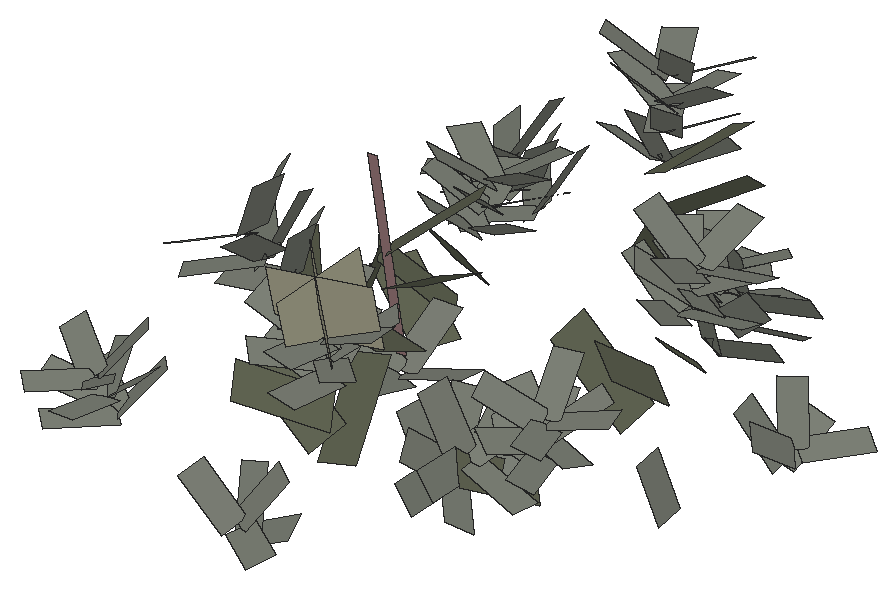
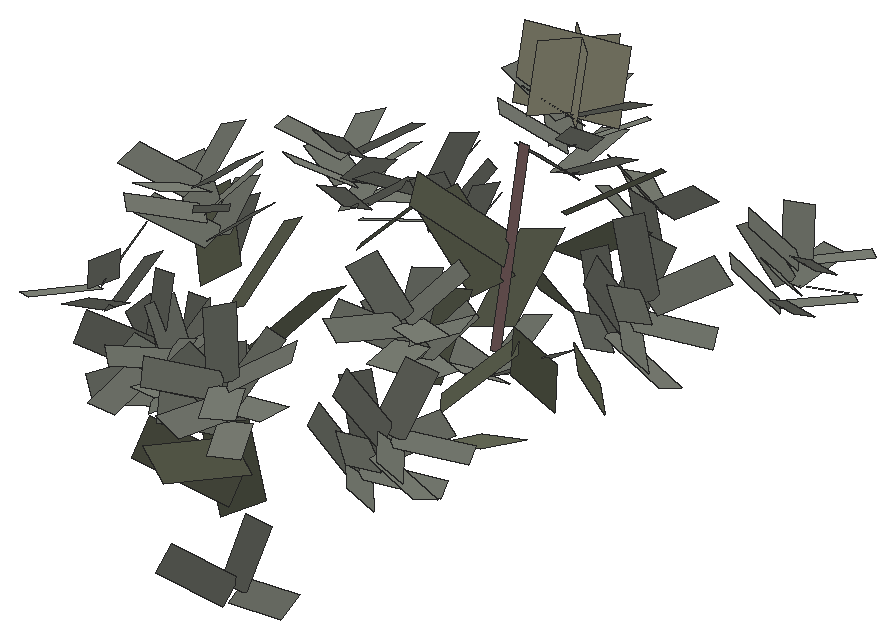
# SketchUp Ruby script. Lengths in inches.
U = 1.inch
M = Sketchup.active_model
def pt(a) = Geom::Point3d.new(a.map { |v| v * U })
def face(e, loops, mat)
  f = e.add_face(loops[0].map { |a| pt(a) })
  loops[1..].each { |l| e.add_face(l.map { |a| pt(a) }).erase! }
  f.material = f.back_material = mat if mat
  f
end
# faces: each face lists its corners as indices into pts; further lists are holes
def faces(e, pts, list, mat = nil) = list.each { |f| face(e, (f[0].is_a?(Array) ? f : [f]).map { |l| l.map { |i| pts[i] } }, mat) }
# xy, xz, yz: faces in a plane at the given z, y or x. An outline is a flat list of corners, or four numbers for a rectangle; further outlines are holes
def ring(l) = l.size == 4 ? [[l[0], l[1]], [l[2], l[1]], [l[2], l[3]], [l[0], l[3]]] : l.each_slice(2).to_a
def flat(e, list, mat, &to3) = list.each { |f| face(e, (f[0].is_a?(Array) ? f : [f]).map { |l| ring(l).map { |u, v| to3.(u, v) } }, mat) }
def xy(e, z, list, mat = nil) = flat(e, list, mat) { |x, y| [x, y, z] }
def xz(e, y, list, mat = nil) = flat(e, list, mat) { |x, z| [x, y, z] }
def yz(e, x, list, mat = nil) = flat(e, list, mat) { |y, z| [x, y, z] }
def lines(e, pts, list) = list.each { |a, b| e.add_line(pt(pts[a]), pt(pts[b])) }
# prism: a flat outline (further loops are holes) pulled along v
def prism(e, loops, v, mat = nil)
  f = face(e, loops, mat); d = Geom::Vector3d.new(v.map { |x| x * U })
  f.pushpull(f.normal.samedirection?(d) ? d.length : -d.length)
end
def box(e, o, s, mat = nil) = prism(e, [[o, [o[0] + s[0], o[1], o[2]], [o[0] + s[0], o[1] + s[1], o[2]], [o[0], o[1] + s[1], o[2]]]], [0, 0, s[2]], mat)
def at(x, y, z, deg = 0) = Geom::Transformation.translation(pt([x, y, z])) * Geom::Transformation.rotation(ORIGIN, Z_AXIS, deg.degrees)
def axes(o, x, y, z) = Geom::Transformation.new([*x, 0, *y, 0, *z, 0, *pt(o).to_a, 1])
def part(name) = M.definitions.add(name)
# library, detail: a bought-in or finely detailed component or shape, given as its bounding box
def library(name, o, s) = part(name).tap { |d| box(d.entities, o, s) }
def detail(e, o, s) = box(e.add_group.entities, o, s)
def put(e, d, t, mat = nil) = e.add_instance(d, t).tap { |i| i.material = mat if mat }
def group(e, t, mat = nil) = e.add_group.tap { |g| g.transformation = t; g.material = mat if mat }.entities
root = M.entities
M.materials.add("tak1dsfasd0f156w").color = [150, 118, 119]
M.materials.add("viburnumblaasdfas0df1w06d").color = [98, 102, 84]
M.materials.add("viburnumbladsadfasdfad0w122").color = [125, 129, 119]
M.materials.add("viburnumbloem2asdfas01vxc5016").color = [175, 173, 148]
c1 = part("Component\#315")
p = [[0.25,0,0],[2.05,0.01,0.35],[1.81,4.2,1.66],[0,4.19,1.3125]]
faces(c1.entities,p,[[0,1,2,3]],"viburnumbladsadfasdfad0w122")
c2 = part("viburnumblad2")
put(c2.entities,c1,axes([-19.23,-4.49,-32.18],[83.35428,0,0],[0,79.38502,0],[0,0,83.35428]))
c3 = part("Component\#314")
p = [[0.14,0,0],[2.58,0.05,0.25],[2.44,5.11,2.64],[0,5.05,2.39]]
faces(c3.entities,p,[[0,1,2,3]],"viburnumblaasdfas0df1w06d")
c4 = part("viburnumblad1\#2")
put(c4.entities,c3,axes([-37.25,6.23,19.31],[75.98784,0,0],[0,65.50676,0],[0,0,75.98784]))
c5 = part("Component\#336")
p = [[6.03,1.45,4.43],[5.85,2.68,0.17],[0,1.22,0],[0.18,0,4.25]]
faces(c5.entities,p,[[0,1,2,3]],"viburnumbloem2asdfas01vxc5016")
c6 = part("Component\#334")
p = [[0.16,3.84,5.17],[0,4.97,1.27],[3.78,1.125,0],[3.9375,0,3.9]]
faces(c6.entities,p,[[0,1,2,3]],"viburnumbloem2asdfas01vxc5016")
c7 = part("Component\#335")
p = [[1.35,5.21,5.35],[1.19,6.33,1.45],[0,1.125,0],[0.16,0,3.9]]
faces(c7.entities,p,[[0,1,2,3]],"viburnumbloem2asdfas01vxc5016")
c8 = part("Component\#337")
p = [[0.6,0,12.07],[1.51,1.22,0.03],[0.91,1.23,0],[0,0,12.04]]
faces(c8.entities,p,[[0,1,2,3]],"tak1dsfasd0f156w")
put(root,c2,axes([2210.91,246.79,41.88],[-0.00636,-0.00796,-0.00575],[0.0099,-0.00571,-0.00294],[-0.00097,-0.00646,0.0087]))
put(root,c2,axes([2209.49,245.54,40.99],[0.00636,0.00796,0.00575],[-0.00984,0.00398,0.00495],[0.00146,-0.00765,0.00773]))
put(root,c2,axes([2209.42,246.71,41.875],[0.00995,-0.00489,-0.00397],[0.00634,0.00703,0.00672],[-0.00053,-0.00802,0.00751]))
put(root,c2,axes([2209.95,247.92,40.99],[0.00254,-0.00908,-0.00688],[0.01053,0.00118,0.00207],[-0.00116,-0.00732,0.00806]))
put(root,c2,axes([2209.29,246.93,40.29],[0.01153,0.00217,0.00126],[-0.00261,0.00855,0.00823],[0.00055,-0.00816,0.00738]))
put(root,c2,axes([2197.875,249.31,44.43],[-0.00773,0.00806,0.00054],[-0.00787,-0.00734,-0.00302],[-0.00183,-0.00247,0.01075]))
put(root,c2,axes([2198.58,250.46,43.45],[-0.01083,0.00076,-0.00267],[-0.00024,-0.01097,-0.00215],[-0.00276,-0.00202,0.01064]))
put(root,c2,axes([2198.09,250.62,44.91],[-0.00759,-0.00699,-0.00431],[0.00733,-0.00841,0.00072],[-0.00369,-0.00233,0.01029]))
put(root,c2,axes([2198.58,250.47,41.96],[-0.00742,0.00774,0.00052],[-0.0085,-0.00793,-0.00326],[-0.00183,-0.00247,0.01075]))
put(root,c2,axes([2197.65,249.76,42.95],[-0.0001,0.01064,0.00343],[-0.01164,0.00037,-0.00146],[-0.00143,-0.00341,0.01055]))
put(root,c2,axes([2197.74,251.62,43.6],[0.0001,-0.01064,-0.00343],[0.01052,-0.00118,0.00394],[-0.00407,-0.00322,0.0099]))
put(root,c2,axes([2211.68,253.05,50.16],[-0.01255,0.00027,0.0006],[-0.00036,-0.0124,-0.00196],[0.00055,-0.00198,0.01239]))
put(root,c2,axes([2196.52,249.63,44.17],[0.00759,0.00699,0.00431],[-0.00801,0.0076,0.00179],[-0.00181,-0.0043,0.01016]))
put(root,c2,axes([2196.74,250.94,44.66],[0.00773,-0.00806,-0.00054],[0.0072,0.00653,0.00553],[-0.00368,-0.00417,0.0097]))
put(root,c2,axes([2196.68,250.64,42.96],[0.01083,-0.00076,0.00267],[-0.0004,0.00932,0.00428],[-0.00274,-0.00461,0.00981]))
put(root,c2,axes([2211.3,254.2,47.23],[-0.01204,0.00026,0.00058],[-0.00039,-0.0134,-0.00212],[0.00055,-0.00198,0.01239]))
put(root,c2,axes([2211.14,253.03,48.49],[-0.00857,0.00873,0.00287],[-0.00949,-0.00914,-0.00056],[0.00162,-0.00243,0.01222]))
put(root,c2,axes([2197.19,250.67,41.69],[0.00793,0.00729,0.0045],[-0.00721,0.00684,0.00161],[-0.00181,-0.0043,0.01016]))
put(root,c2,axes([2197.3,251.77,42.17],[0.00743,-0.00696,-0.00145],[0.0072,0.00653,0.00553],[-0.00282,-0.00502,0.00959]))
put(root,c2,axes([2211.3125,254.38,48.9],[-0.00917,-0.00834,-0.00202],[0.00857,-0.00908,-0.00138],[-0.00054,-0.00239,0.01232]))
put(root,c4,axes([2210.54,254.06,43.96],[-0.00623,0.01061,0.0062],[-0.01365,-0.00831,0.0005],[0.00356,-0.0051,0.0123]))
put(root,c5,axes([2207.86,251.38,49.92],[1.0472,0,0],[0,1.0472,0],[0,0,1.0472]))
put(root,c6,axes([2208.61,250.23,49.61],[1.0472,0,0],[0,1.0472,0],[0,0,1.0472]))
put(root,c2,axes([2210.35,252.2,49.97],[0.00042,0.01207,0.00346],[-0.01239,-0.00016,0.00207],[0.00203,-0.00348,0.0119]))
put(root,c7,axes([2210.11,249.6,49.53],[1.0472,0,0],[0,1.0472,0],[0,0,1.0472]))
put(root,c2,axes([2210.81,254.32,50.5625],[-0.00042,-0.01207,-0.00346],[0.01251,-0.00069,0.00087],[-0.00103,-0.00342,0.01205]))
put(root,c2,axes([2218.88,255.93,43.26],[-0.00894,0.00051,0.00882],[-0.00128,-0.01248,-0.00058],[0.00874,-0.00131,0.00893]))
put(root,c2,axes([2210.04,253.22,47.05],[0.00044,0.0126,0.00361],[-0.01115,-0.00014,0.00186],[0.00203,-0.00348,0.0119]))
put(root,c2,axes([2209.66,252.96,48.52],[0.00917,0.00834,0.00202],[-0.00775,0.00756,0.00397],[0.00155,-0.00451,0.01162]))
put(root,c2,axes([2216.625,256.45,41.18],[-0.00933,0.00053,0.0092],[-0.00115,-0.01124,-0.00052],[0.00874,-0.00131,0.00893]))
put(root,c2,axes([2217.64,257.13,42.53],[-0.00797,-0.00829,0.00506],[0.00596,-0.00975,-0.0066],[0.00788,-0.0017,0.00963]))
put(root,c2,axes([2217.44,255.69,42.25],[-0.00467,0.00901,0.00741],[-0.00631,-0.00787,0.00559],[0.00942,-0.00179,0.00811]))
put(root,c4,axes([2209.14,254.43,41.85],[0.00552,0.01118,0.00587],[-0.01458,0.00491,0.00435],[0.00124,-0.00686,0.01189]))
put(root,c2,axes([2209.48,253.47,50.375],[0.01255,-0.00027,-0.0006],[0.00048,0.01156,0.0049],[0.00045,-0.00492,0.01155]))
put(root,c2,axes([2209.73,254.65,49.04],[0.00857,-0.00873,-0.00287],[0.00926,0.00794,0.00351],[-0.00062,-0.00447,0.01173]))
put(root,c2,axes([2217.79,255.09,44.05],[0.00233,0.01223,0.00166],[-0.00783,0.00016,0.00982],[0.00954,-0.00286,0.00766]))
put(root,c2,axes([2209.25,254.24,47.47],[0.01143,0.00024,-0.0017],[0.00048,0.01156,0.0049],[0.0018,-0.00492,0.01142]))
put(root,c2,axes([2218.47,257.23,44.07],[-0.00233,-0.01223,-0.00166],[0.00991,-0.00085,-0.00768],[0.00736,-0.00274,0.0098]))
put(root,c2,axes([2215.78,255.66,41.89],[0.00119,0.01147,0.00076],[-0.00783,0.00016,0.00982],[0.00974,-0.00152,0.00779]))
put(root,c2,axes([2222.57,258.84,46.21],[-0.01096,-0.00354,0.00194],[0.00316,-0.01102,-0.00224],[0.00251,-0.00157,0.0113]))
put(root,c2,axes([2221.92,258.67,44.73],[-0.00975,0.0051,0.00392],[-0.00563,-0.0109,0.00018],[0.00356,-0.00165,0.01101]))
put(root,c4,axes([2220.57,259.39,40.65],[-0.00789,0.00746,0.00681],[-0.00938,-0.01142,0.00165],[0.00606,-0.00342,0.01077]))
put(root,c2,axes([2221.56,259.74,43.59],[-0.01053,-0.0034,0.00186],[0.00341,-0.01191,-0.00242],[0.00251,-0.00157,0.0113]))
put(root,c2,axes([2216.2,255.76,43.52],[0.00797,0.00829,-0.00506],[-0.00363,0.00868,0.00851],[0.00902,-0.0039,0.00783]))
put(root,c2,axes([2221.65,257.69,46.15],[-0.00283,0.01075,0.0036],[-0.01053,-0.00387,0.00326],[0.00419,-0.00245,0.01063]))
put(root,c2,axes([2216.68,257.3,43.5625],[0.00467,-0.00901,-0.00741],[0.00895,0.00789,-0.00395],[0.00748,-0.00381,0.00935]))
put(root,c2,axes([2217.38,256.39,44.86],[0.00894,-0.00051,-0.00882],[0.00335,0.0118,0.00272],[0.00817,-0.00429,0.00853]))
put(root,c2,axes([2221.71,259.91,45.14],[-0.00575,-0.0101,-0.00117],[0.01003,-0.00542,-0.00255],[0.00167,-0.00226,0.01134]))
put(root,c4,axes([2208.125,256.4,39.75],[0.0147,-0.00029,0.00242],[-0.00086,0.01575,0.00709],[-0.00232,-0.00615,0.01338]))
put(root,c2,axes([2220.74,258.5,43.52],[-0.00295,0.01122,0.00376],[-0.00948,-0.00348,0.00294],[0.00419,-0.00245,0.01063]))
put(root,c2,axes([2221.48,259.69,46.72],[0.00283,-0.01075,-0.0036],[0.01123,0.00316,-0.00059],[0.00152,-0.00332,0.0111]))
put(root,c2,axes([2220.65,258.16,44.91],[0.00575,0.0101,0.00117],[-0.00857,0.00432,0.00479],[0.00404,-0.00351,0.01039]))
put(root,c2,axes([2220.56,258.55,46.66],[0.01096,0.00354,-0.00194],[-0.00246,0.01032,0.00491],[0.0032,-0.00419,0.01042]))
put(root,c2,axes([2220.27,259.66,45.45],[0.00975,-0.0051,-0.00392],[0.00612,0.00977,0.00252],[0.00215,-0.00412,0.01072]))
put(root,c2,axes([2219.79,259.16,44.04],[0.00971,0.00365,-0.00281],[-0.00246,0.01032,0.00491],[0.00437,-0.00379,0.01015]))
put(root,c2,axes([2198.02,262.85,48.33],[-0.00996,0.00362,-0.00815],[-0.00316,-0.01285,-0.00186],[-0.00834,0.00054,0.01043]))
put(root,c2,axes([2199.18,264.05,47.21],[-0.00854,-0.00651,-0.00796],[0.00449,-0.01178,0.00482],[-0.00927,0.0004,0.00962]))
put(root,c4,axes([2207.59,265.23,42.92],[-0.0155,-0.00126,0.00308],[0.00163,-0.01831,0.00072],[0.00301,0.00088,0.01554]))
put(root,c2,axes([2198.72,262.5,46.66],[-0.00554,0.01163,-0.00356],[-0.00953,-0.00658,-0.00667],[-0.00756,-0.00023,0.01102]))
put(root,c2,axes([2226.6,262.48,39.98],[-0.00142,0.01147,0.00174],[-0.00575,-0.00222,0.00993],[0.01007,0.00035,0.00591]))
put(root,c2,axes([2197.51,264.4375,48.06],[-0.00212,-0.01282,-0.00311],[0.00883,-0.00372,0.00932],[-0.00981,-0.00058,0.00906]))
put(root,c2,axes([2207.35,265.27,40.98],[-0.01323,-0.00019,0.0019],[0.00023,-0.01336,0.00026],[0.00189,0.00029,0.01323]))
put(root,c2,axes([2199.55,264.8125,45.62],[-0.00096,-0.01167,-0.00375],[0.00883,-0.00372,0.00932],[-0.00998,-0.00196,0.00867]))
put(root,c2,axes([2199.27,262.74,44.98],[0.00203,0.01231,0.00299],[-0.01181,0.00375,-0.0074],[-0.00738,-0.00146,0.01104]))
put(root,c8,axes([2205.03,263.99,42.22],[1.0472,0,0],[0,1.0472,0],[0,0,1.0472]))
put(root,c2,axes([2197.8,264.57,46.03],[0.00554,-0.01163,0.00356],[0.00681,0.00581,0.00839],[-0.00964,-0.00181,0.00908]))
put(root,c4,axes([2206.57,266.31,45.8125],[-0.00531,-0.01357,0.00158],[0.01582,-0.00598,0.00178],[-0.00086,0.00203,0.01449]))
put(root,c2,axes([2205.98,264.28,41.08],[0,0.0133,0.00135],[-0.0129,-0.00035,0.00349],[0.0035,-0.0013,0.01283]))
put(root,c2,axes([2197.64,263.03,45.75],[0.00854,0.00651,0.00796],[-0.00689,0.01199,-0.00242],[-0.00792,-0.00244,0.01048]))
put(root,c2,axes([2196.33,263.88,46.99],[0.00996,-0.00362,0.00815],[0.00104,0.0126,0.00432],[-0.00886,-0.00258,0.00967]))
put(root,c2,axes([2206.38,266.625,41.26],[0,-0.0133,-0.00135],[0.01336,0.00003,-0.00028],[0.00028,-0.00135,0.01329]))
put(root,c2,axes([2198.63,264.28,44.64],[0.01039,-0.00378,0.00851],[0.00094,0.01134,0.00389],[-0.00886,-0.00258,0.00967]))
put(root,c4,axes([2200.69,263.9,41.91],[0.00849,0.00329,0.01149],[-0.00585,0.01597,-0.00025],[-0.01083,-0.00383,0.0091]))
put(root,c4,axes([2205.18,265.79,48.1],[0.00718,-0.01267,0.00168],[0.01433,0.00855,0.00326],[-0.00327,0.00004,0.01429]))
put(root,c4,axes([2202.2,265.49,40.29],[0.00719,-0.00894,0.00913],[0.00526,0.01343,0.009],[-0.01194,-0.00098,0.00844]))
put(root,c2,axes([2205.02,265.64,41.35],[0.01323,0.00019,-0.0019],[0.00023,0.01303,0.00294],[0.00189,-0.00295,0.0129]))
put(root,c4,axes([2220.42,270.45,41.85],[-0.01118,0.00552,0.00587],[-0.00491,-0.01458,0.00435],[0.00686,0.00124,0.01189]))
put(root,c4,axes([2220.79,271.85,43.96],[-0.01061,-0.00623,0.0062],[0.00831,-0.01365,0.0005],[0.0051,0.00356,0.0123]))
put(root,c2,axes([2221.63,271.35,47.05],[-0.0126,0.00044,0.00361],[0.00014,-0.01115,0.00186],[0.00348,0.00203,0.0119]))
put(root,c2,axes([2229.3125,270.79,40.99],[-0.00796,0.00636,0.00575],[-0.00398,-0.00984,0.00495],[0.00765,0.00146,0.00773]))
put(root,c2,axes([2222.65,271.66,49.97],[-0.01207,0.00042,0.00346],[0.00016,-0.01239,0.00207],[0.00348,0.00203,0.0119]))
put(root,c4,axes([2218.45,269.43,39.75],[0.00029,0.0147,0.00242],[-0.01575,-0.00086,0.00709],[0.00615,-0.00232,0.01338]))
put(root,c4,axes([2205.79,270.6,41.71],[-0.00837,0.01093,-0.00027],[-0.01213,-0.00903,0.00454],[0.00324,0.00308,0.01192]))
put(root,c2,axes([2221.89,270.97,48.52],[-0.00834,0.00917,0.00202],[-0.00756,-0.00775,0.00397],[0.00451,0.00155,0.01162]))
put(root,c2,axes([2221.82,272.45,48.49],[-0.00873,-0.00857,0.00287],[0.00914,-0.00949,-0.00056],[0.00243,0.00162,0.01222]))
put(root,c4,axes([2206.21,272.46,43.3],[-0.0135,0.00082,0.00242],[0.00046,-0.01443,0.00598],[0.00274,0.00585,0.01119]))
put(root,c2,axes([2227.92,270.6,40.29],[-0.00217,0.01153,0.00126],[-0.00855,-0.00261,0.00823],[0.00816,0.00055,0.00738]))
put(root,c2,axes([2220.61,270.56,47.47],[-0.00024,0.01143,-0.0017],[-0.01156,0.00048,0.0049],[0.00492,0.0018,0.01142]))
put(root,c2,axes([2221.39,270.79,50.375],[0.00027,0.01255,-0.0006],[-0.01156,0.00048,0.0049],[0.00492,0.00045,0.01155]))
put(root,c2,axes([2220.65,272.6,47.23],[-0.00026,-0.01204,0.00058],[0.0134,-0.00039,-0.00212],[0.00198,0.00055,0.01239]))
put(root,c4,axes([2204.2,269.65,39.48],[0.00652,0.01335,-0.00071],[-0.01553,0.00758,0.00028],[0.00058,0.00086,0.01356]))
put(root,c2,axes([2205.86,272.9,46.21],[-0.01136,0.00626,-0.00167],[-0.00561,-0.00886,0.00368],[0.00077,0.00497,0.01057]))
put(root,c2,axes([2221.8,272.99,50.16],[-0.00027,-0.01255,0.0006],[0.0124,-0.00036,-0.00196],[0.00198,0.00055,0.01239]))
put(root,c2,axes([2228.14,270.73,41.875],[0.00489,0.00995,-0.00397],[-0.00703,0.00634,0.00672],[0.00802,-0.00053,0.00751]))
put(root,c2,axes([2206.16,274.32,47.25],[-0.01214,-0.0031,0.00083],[0.00339,-0.01158,0.00463],[-0.0004,0.00512,0.01053]))
put(root,c2,axes([2206.1,273.9,48.91],[-0.01088,0.00599,-0.0016],[-0.00623,-0.00984,0.00409],[0.00077,0.00497,0.01057]))
put(root,c2,axes([2205.58,274.39,45.78],[-0.00603,-0.00996,0.00266],[0.01166,-0.00593,0.00316],[-0.00133,0.00444,0.01071]))
put(root,c2,axes([2220.2,271.04,49.04],[0.00873,0.00857,-0.00287],[-0.00794,0.00926,0.00351],[0.00447,-0.00062,0.01173]))
put(root,c2,axes([2226.93,271.26,40.99],[0.00908,0.00254,-0.00688],[-0.00118,0.01053,0.00207],[0.00732,-0.00116,0.00806]))
put(root,c2,axes([2228.0625,272.22,41.88],[0.00796,-0.00636,-0.00575],[0.00571,0.0099,-0.00294],[0.00646,-0.00097,0.0087]))
put(root,c2,axes([2220.47,272.62,48.9],[0.00834,-0.00917,-0.00202],[0.00908,0.00857,-0.00138],[0.00239,-0.00054,0.01232]))
put(root,c2,axes([2205.52,273.04,47.58],[-0.00325,0.01157,-0.00309],[-0.01106,-0.00241,0.00198],[0.00148,0.00409,0.01081]))
put(root,c2,axes([2205.96,275.41,48.5],[-0.00628,-0.01038,0.00277],[0.0108,-0.00549,0.00293],[-0.00133,0.00444,0.01071]))
put(root,c2,axes([2220.53,272.12,50.5625],[0.01207,-0.00042,-0.00346],[0.00069,0.01251,0.00087],[0.00342,-0.00103,0.01205]))
put(root,c2,axes([2204.53,272.75,46.35],[0.00561,0.0092,-0.00364],[-0.0108,0.0064,-0.00025],[0.002,0.00408,0.01074]))
put(root,c2,axes([2205,275.1,47.07],[0.00325,-0.01157,0.00309],[0.01204,0.00353,0.00052],[-0.00148,0.00333,0.01101]))
put(root,c2,axes([2204.52,273.77,48.94],[0.00628,0.01038,-0.00277],[-0.0108,0.0064,-0.00025],[0.00133,0.00298,0.0111]))
put(root,c2,axes([2203.99,273.9,47.38],[0.01214,0.0031,-0.00083],[-0.00326,0.01206,-0.00174],[0.0004,0.0023,0.01128]))
put(root,c2,axes([2219.19,277.09,41.89],[-0.01147,0.00119,0.00076],[-0.00016,-0.00783,0.00982],[0.00152,0.00974,0.00779]))
put(root,c2,axes([2204.38,275.27,48.54],[0.01088,-0.00599,0.0016],[0.00623,0.01076,-0.00141],[-0.00077,0.00244,0.01124]))
put(root,c2,axes([2218.4,277.93,41.18],[-0.00053,-0.00933,0.0092],[0.01124,-0.00115,-0.00052],[0.00131,0.00874,0.00893]))
put(root,c2,axes([2219.16,278.75,42.25],[-0.00901,-0.00467,0.00741],[0.00787,-0.00631,0.00559],[0.00179,0.00942,0.00811]))
put(root,c2,axes([2219.09,277.51,43.52],[-0.00829,0.00797,-0.00506],[-0.00868,-0.00363,0.00851],[0.0039,0.00902,0.00783]))
put(root,c2,axes([2216.69,278.43,42.43],[-0.00726,0.00696,-0.0015],[-0.00749,-0.00689,0.00431],[0.00194,0.00418,0.01005]))
put(root,c2,axes([2216.83,279.55,42.06],[-0.00812,-0.00757,0.00318],[0.00703,-0.00685,0.00164],[0.0009,0.00343,0.01047]))
put(root,c2,axes([2217.23,279.48,43.35],[-0.0109,0.00051,0.00178],[0.00012,-0.00953,0.00349],[0.00185,0.00377,0.01023]))
put(root,c2,axes([2219.76,279.1,44.05],[-0.01223,0.00233,0.00166],[-0.00016,-0.00783,0.00982],[0.00286,0.00954,0.00766]))
put(root,c2,axes([2217.03,279.05,44.98],[-0.00764,0.00797,-0.00053],[-0.00749,-0.00689,0.00431],[0.00278,0.00334,0.01017]))
put(root,c2,axes([2217.27,280.38,44.63],[-0.00778,-0.00725,0.00304],[0.00781,-0.00761,0.00182],[0.0009,0.00343,0.01047]))
put(root,c2,axes([2202.85,280.37,44.97],[-0.00962,0.00434,-0.00682],[-0.00417,-0.01174,-0.00159],[-0.00692,0.00104,0.01043]))
put(root,c2,axes([2201.98,281.01,46.33],[-0.00913,-0.00526,-0.00683],[0.00354,-0.01136,0.00402],[-0.00787,0.001,0.00974]))
put(root,c2,axes([2216.14,278.47,43.81],[0.0001,0.01076,-0.00253],[-0.0107,0.00082,0.00309],[0.00316,0.0024,0.01032]))
put(root,c2,axes([2201.36,279.63,45.83],[-0.00447,0.0114,-0.0028],[-0.00996,-0.00527,-0.00554],[-0.00621,0.00025,0.01092]))
put(root,c2,axes([2217.72,278.95,42.53],[0.00829,-0.00797,0.00506],[0.00975,0.00596,-0.0066],[0.0017,0.00788,0.00963]))
put(root,c2,axes([2216.26,280.35,43.33],[-0.0001,-0.01076,0.00253],[0.0116,-0.00022,-0.00049],[0.00051,0.00252,0.01075]))
put(root,c2,axes([2218.92,280.19,43.26],[-0.00051,-0.00894,0.00882],[0.01248,-0.00128,-0.00058],[0.00131,0.00874,0.00893]))
put(root,c2,axes([2203.32,280.09,43.38],[-0.00429,0.01094,-0.00269],[-0.01076,-0.0057,-0.00599],[-0.00621,0.00025,0.01092]))
put(root,c2,axes([2217.55,277.98,43.5625],[0.00901,0.00467,-0.00741],[-0.00789,0.00895,-0.00395],[0.00381,0.00748,0.00935]))
put(root,c2,axes([2218.46,278.6875,44.86],[0.00051,0.00894,-0.00882],[-0.0118,0.00335,0.00272],[0.00429,0.00817,0.00853]))
put(root,c2,axes([2202.46,281.92,44.74],[-0.0033,-0.01178,-0.00285],[0.00874,-0.0044,0.00808],[-0.00849,0.00014,0.00926]))
put(root,c2,axes([2215.44,279.72,42.22],[0.00733,-0.00766,0.00051],[0.00858,0.00809,-0.00187],[0.00089,0.00157,0.01091]))
put(root,c2,axes([2215.67,279.35,45.15],[0.00778,0.00725,-0.00304],[-0.00736,0.00822,0.00077],[0.00276,0.00149,0.0106]))
put(root,c2,axes([2201.79,279.89,44.15],[0.0033,0.01178,0.00285],[-0.01097,0.00447,-0.0058],[-0.00615,-0.00092,0.01092]))
put(root,c2,axes([2215.32,279.62,43.6875],[0.0109,-0.00051,-0.00178],[0.00032,0.01098,-0.00121],[0.00182,0.00115,0.01084]))
put(root,c2,axes([2215.92,280.68,44.8],[0.00764,-0.00797,0.00053],[0.00794,0.00749,-0.00173],[0.00089,0.00157,0.01091]))
put(root,c2,axes([2217.62,279.78,44.07],[0.01223,-0.00233,-0.00166],[0.00085,0.00991,-0.00768],[0.00274,0.00736,0.0098]))
put(root,c2,axes([2200.85,281.8,45.54],[0.00447,-0.0114,0.0028],[0.00817,0.00518,0.00802],[-0.00843,-0.00103,0.00925]))
put(root,c2,axes([2202.53,281.97,43.05],[0.00493,-0.01032,0.00165],[0.00817,0.00518,0.00802],[-0.0079,-0.00226,0.0095]))
put(root,c2,axes([2200.24,280.43,45.04],[0.00913,0.00526,0.00683],[-0.00534,0.01127,-0.00154],[-0.00678,-0.00178,0.01043]))
put(root,c2,axes([2201.19,281.18,43.74],[0.00962,-0.00434,0.00682],[0.00218,0.01069,0.00373],[-0.00772,-0.00183,0.00974]))
put(root,c2,axes([2202.11,280.77,42.58],[0.00954,0.0055,0.00713],[-0.0048,0.01014,-0.00139],[-0.00678,-0.00178,0.01043]))
put(root,c4,axes([2209.09,284.74,39.45],[-0.01228,-0.00656,0.00533],[0.00976,-0.01204,0.00766],[0.00081,0.00845,0.01225]))
put(root,c2,axes([2208.17,287.22,47.11],[-0.00983,-0.00604,0.00067],[0.00618,-0.00942,0.00556],[-0.00236,0.00509,0.01124]))
put(root,c2,axes([2208.2,286.87,48.76],[-0.01213,0.00288,-0.00157],[-0.00331,-0.01081,0.00577],[-0.00003,0.00592,0.01108]))
put(root,c2,axes([2208.01,288.21,49.94],[-0.01088,-0.00598,0.00194],[0.00618,-0.00942,0.00556],[-0.00119,0.00576,0.0111]))
put(root,c2,axes([2207.34,286.87,50.45],[-0.00627,0.01006,-0.00416],[-0.01085,-0.00538,0.00335],[0.0009,0.00527,0.01137]))
put(root,c4,axes([2207.54,286.26,41.6],[0.00185,-0.01141,0.00751],[0.01551,0.00355,0.00158],[-0.0028,0.0071,0.01148]))
put(root,c2,axes([2207.32,288.28,48.14],[-0.00325,-0.01134,0.00432],[0.011,-0.00211,0.00274],[-0.0019,0.00489,0.01141]))
put(root,c2,axes([2206.7,286.31,48.93],[0.00325,0.01134,-0.00432],[-0.01209,0.00342,-0.00014],[0.00105,0.00419,0.0118]))
put(root,c2,axes([2206.92,287.64,46.79],[0.00655,-0.0105,0.00435],[0.00967,0.00585,-0.00045],[-0.00175,0.00381,0.01184]))
put(root,c2,axes([2206.38,286.22,47.28],[0.01044,0.00574,-0.00186],[-0.00678,0.01138,-0.00292],[0.00034,0.00331,0.01211]))
put(root,c4,axes([2206.47,286.21,43.93],[0.01159,-0.00514,0.00541],[0.00744,0.01388,-0.00276],[-0.00381,0.00452,0.01245]))
put(root,c2,axes([2206.57,288.82,49.65],[0.00627,-0.01006,0.00416],[0.01074,0.0065,-0.0005],[-0.00175,0.00381,0.01184]))
put(root,c2,axes([2206.1,287.49,48.42],[0.01213,-0.00288,0.00157],[0.00334,0.0124,-0.003],[-0.00082,0.00316,0.01213]))
put(root,c2,axes([2205.9,287.47,50.16],[0.01088,0.00598,-0.00194],[-0.00628,0.01054,-0.00271],[0.00034,0.00331,0.01211]))
put(root,c2,axes([2203.39,292.76,41.24],[-0.01151,-0.00126,-0.00215],[-0.00083,-0.00812,0.00826],[-0.00252,0.0083,0.00677]))
put(root,c2,axes([2202.16,291.97,41.55],[0.00052,0.00907,-0.00737],[-0.01174,-0.00037,-0.00119],[-0.00118,0.00734,0.00793]))
put(root,c2,axes([2202.6,293.6,40.32],[-0.00052,-0.00907,0.00737],[0.0111,0.00213,0.00308],[-0.00399,0.00704,0.00741]))
